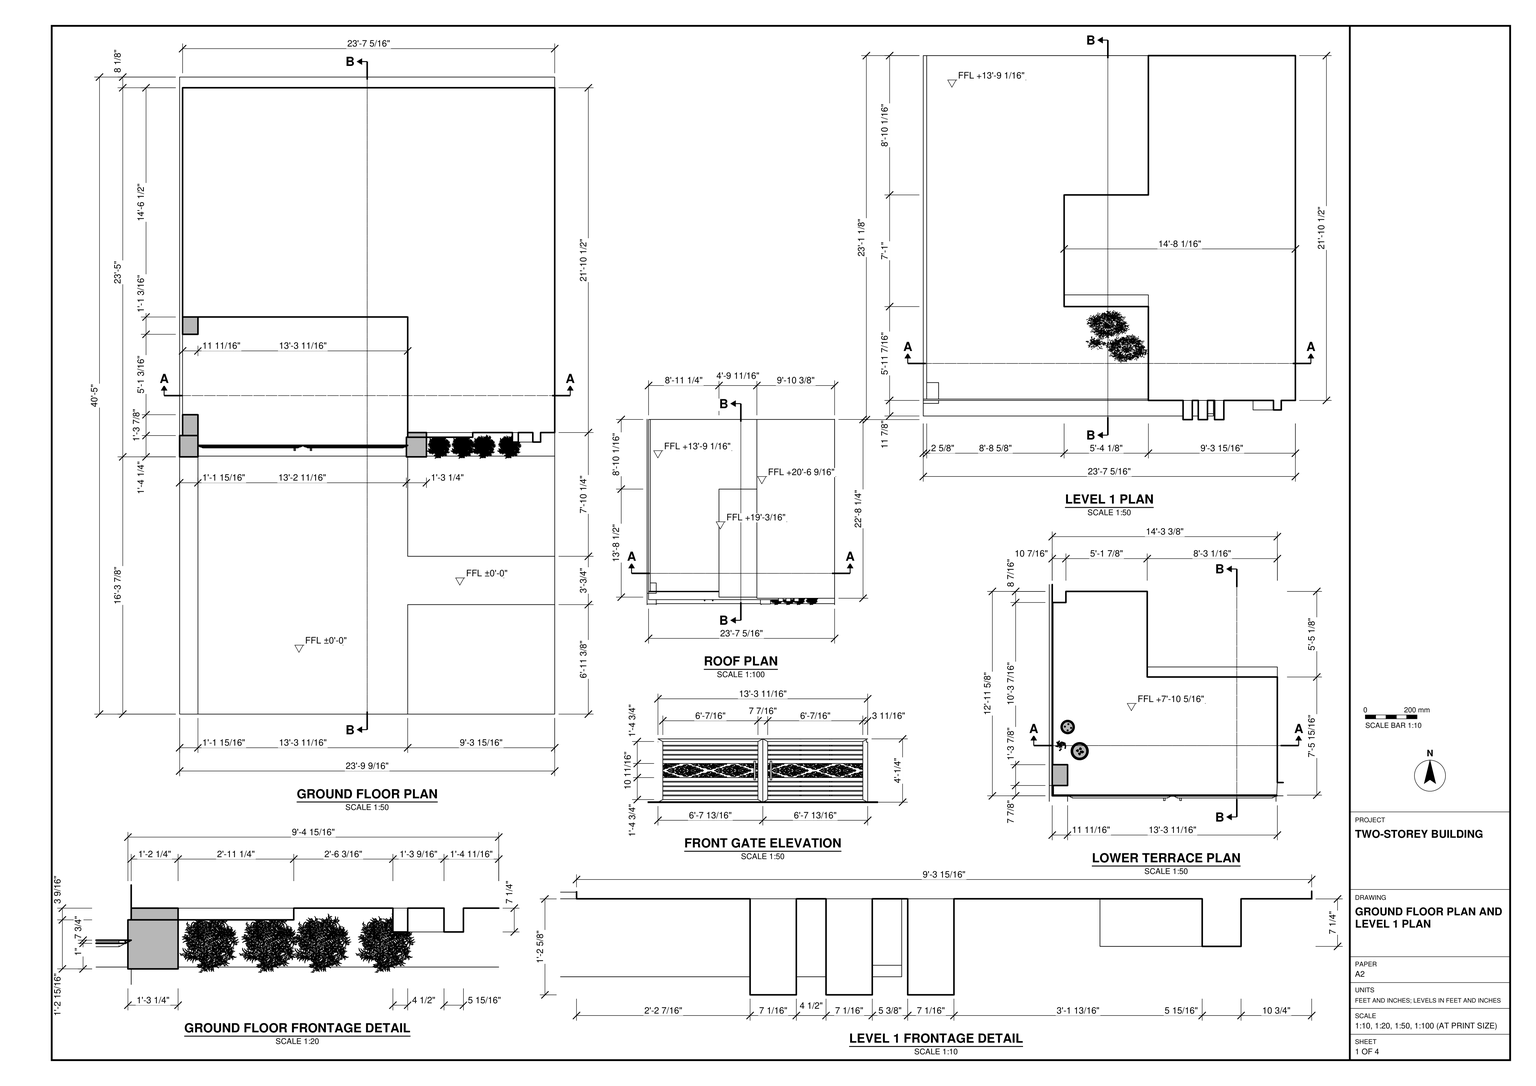
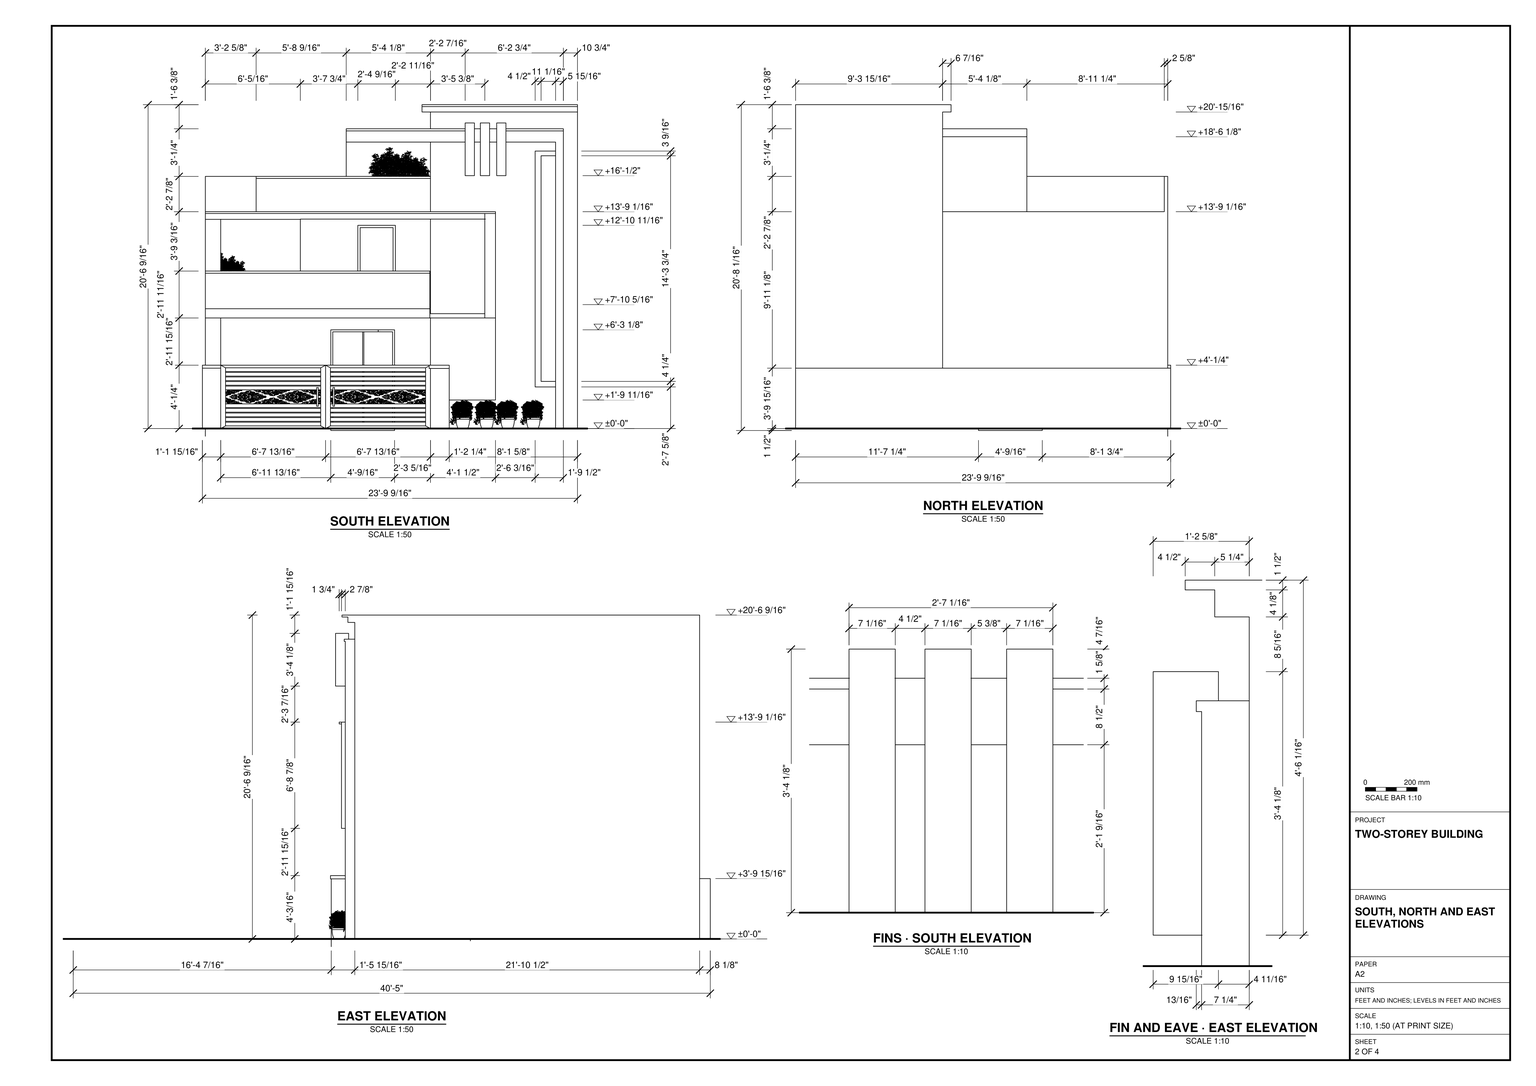
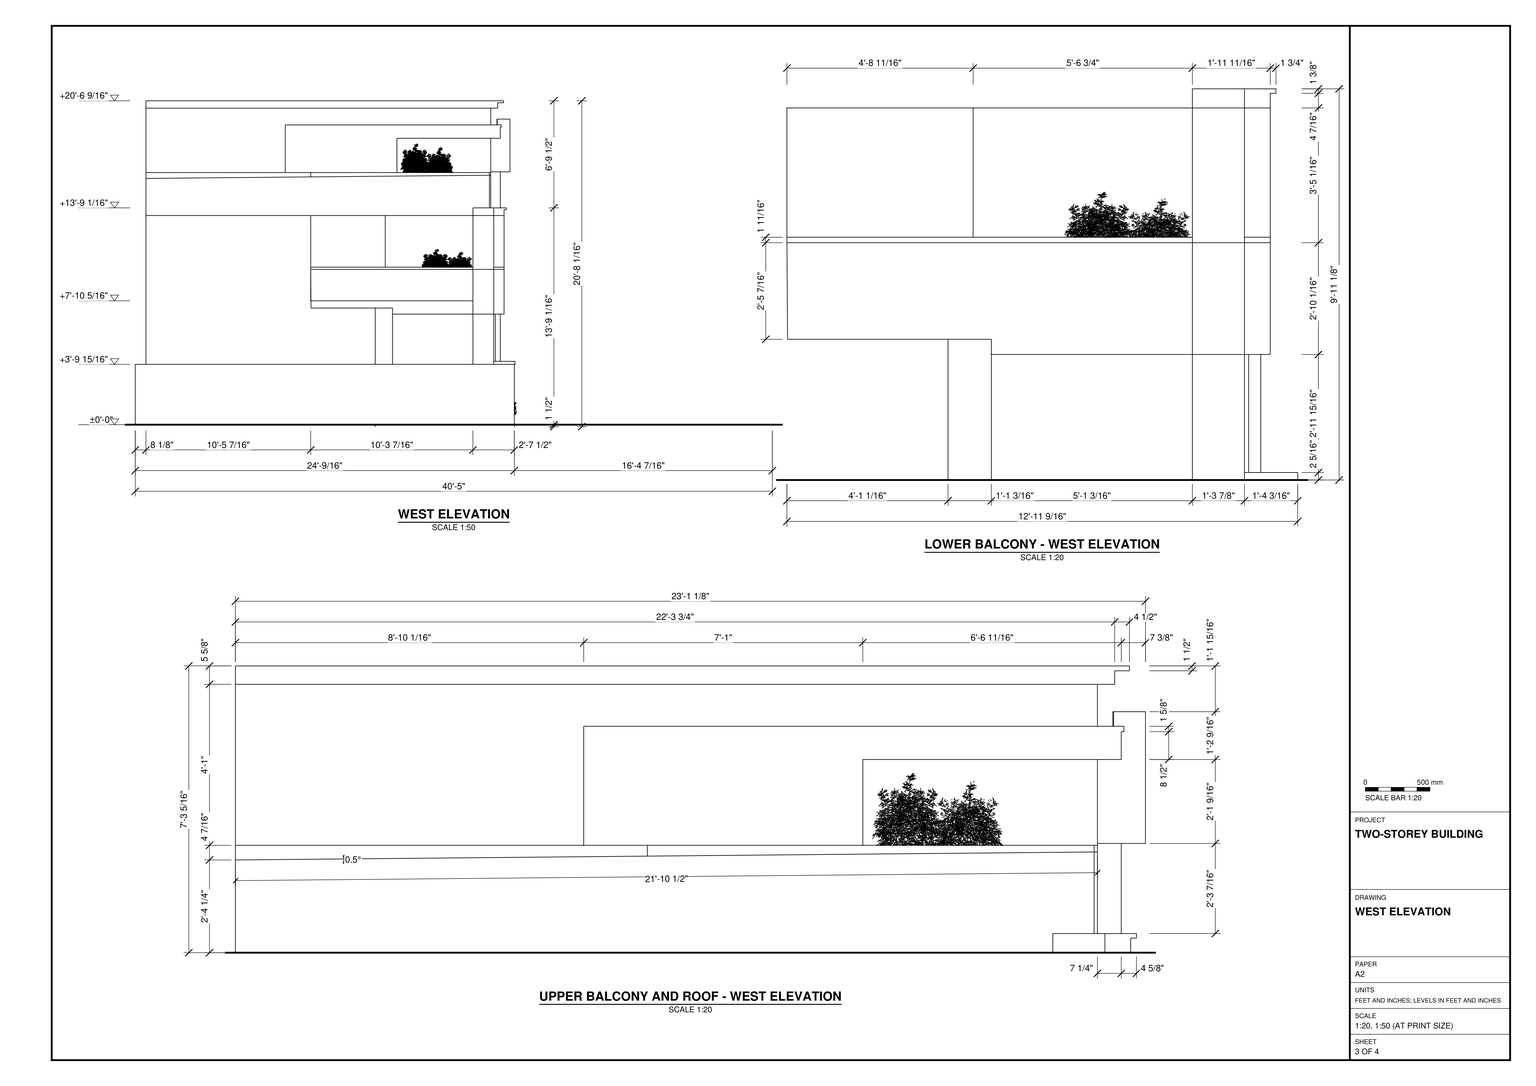
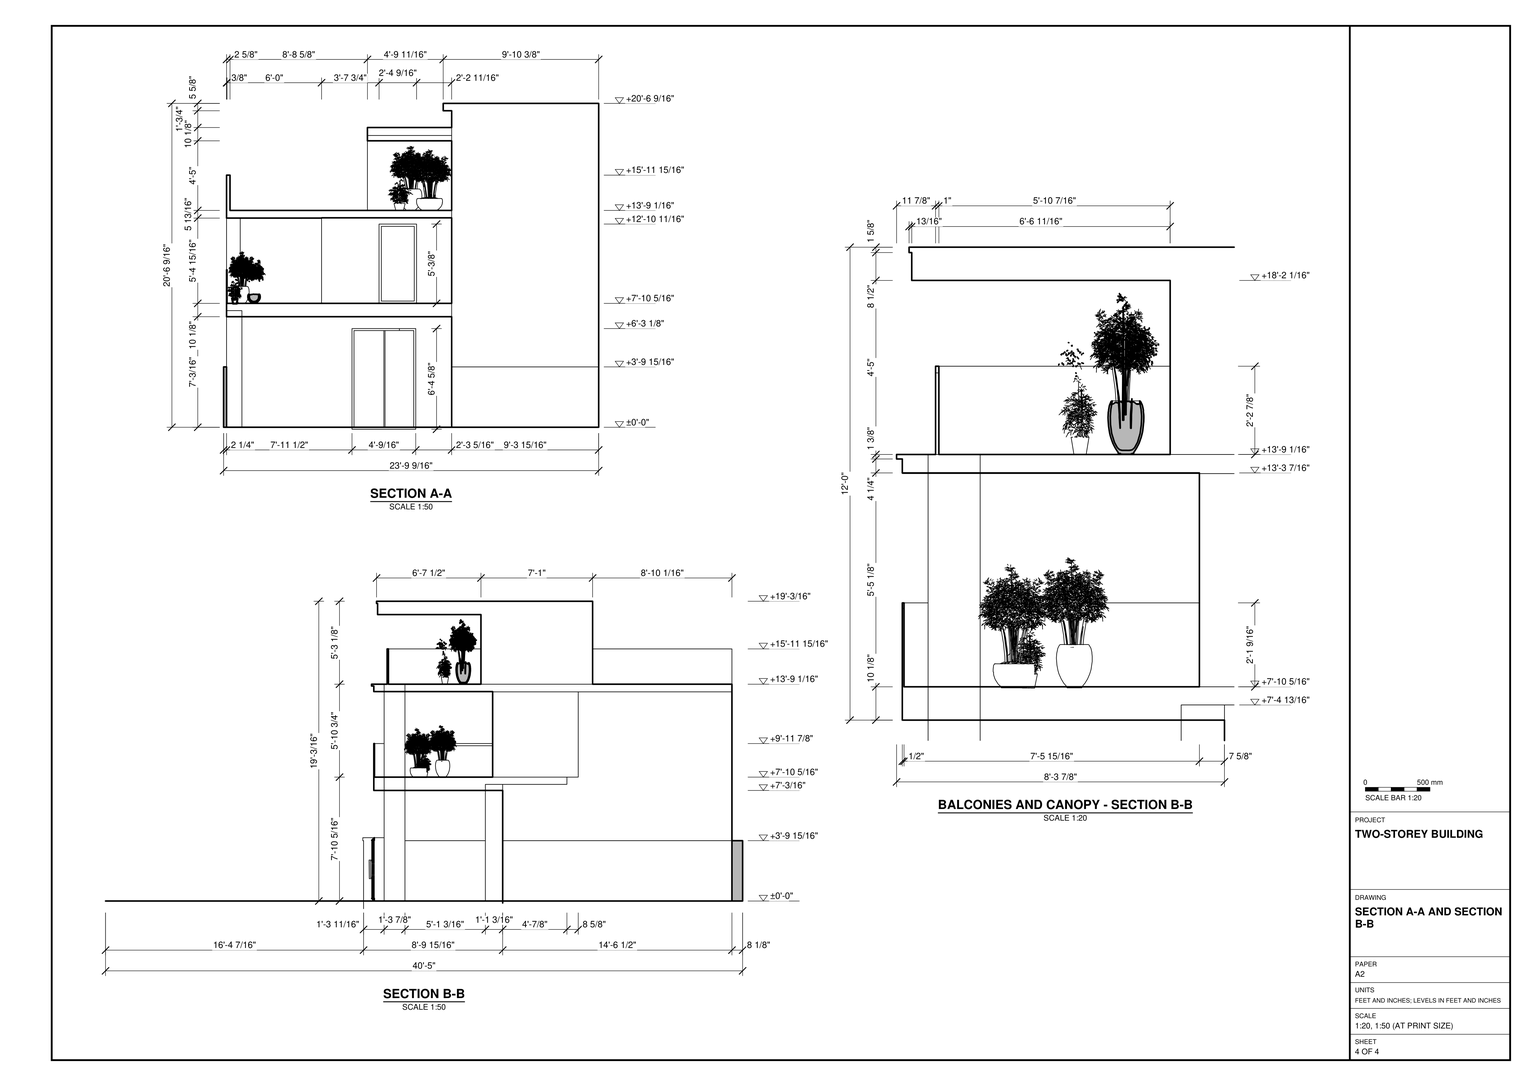
Build the two-storey building and its frontage in SketchUp from task_files/diagram_01.pdf. Work in feet and inches. Including the ground surface in front of the gate, the model must measure 23'-9 9/16" across the frontage, 40'-5" from front to back and 20'-8 1/16" in overall height. Set the ground floor at ±0'-0" and Level 1 at +13'-9 1/16". The lower terrace is between these levels at +7'-10 5/16".

Use the plans to set out the walls, openings, slab edges and terrace recesses. Follow the drawn thicknesses of the walls and parapets. On the south frontage, place the paired gate leaves between posts in front of the open bay, with the row of planters to the right. Use the west elevation to shape the solid balcony fronts and the setbacks between the terraces and flat roof planes. Include the tall frame on the right of the south elevation, its projecting eave and the three vertical fins.

Keep shell elements such as walls, slabs and roof pieces in separate groups or components, and group each furniture or joinery piece separately. Use components for repeated parts. Decor and loose items, including plants, may be any suitable library components. Save one SketchUp model as output_files/two_storey_building_stepped_terraces_and_gated_frontage.skp.

# SketchUp Ruby script. Lengths in inches.
U = 1.inch
M = Sketchup.active_model
def pt(a) = Geom::Point3d.new(a.map { |v| v * U })
def face(e, loops, mat)
  f = e.add_face(loops[0].map { |a| pt(a) })
  loops[1..].each { |l| e.add_face(l.map { |a| pt(a) }).erase! }
  f.material = f.back_material = mat if mat
  f
end
# faces: each face lists its corners as indices into pts; further lists are holes
def faces(e, pts, list, mat = nil) = list.each { |f| face(e, (f[0].is_a?(Array) ? f : [f]).map { |l| l.map { |i| pts[i] } }, mat) }
# xy, xz, yz: faces in a plane at the given z, y or x. An outline is a flat list of corners, or four numbers for a rectangle; further outlines are holes
def ring(l) = l.size == 4 ? [[l[0], l[1]], [l[2], l[1]], [l[2], l[3]], [l[0], l[3]]] : l.each_slice(2).to_a
def flat(e, list, mat, &to3) = list.each { |f| face(e, (f[0].is_a?(Array) ? f : [f]).map { |l| ring(l).map { |u, v| to3.(u, v) } }, mat) }
def xy(e, z, list, mat = nil) = flat(e, list, mat) { |x, y| [x, y, z] }
def xz(e, y, list, mat = nil) = flat(e, list, mat) { |x, z| [x, y, z] }
def yz(e, x, list, mat = nil) = flat(e, list, mat) { |y, z| [x, y, z] }
def lines(e, pts, list) = list.each { |a, b| e.add_line(pt(pts[a]), pt(pts[b])) }
# prism: a flat outline (further loops are holes) pulled along v
def prism(e, loops, v, mat = nil)
  f = face(e, loops, mat); d = Geom::Vector3d.new(v.map { |x| x * U })
  f.pushpull(f.normal.samedirection?(d) ? d.length : -d.length)
end
def box(e, o, s, mat = nil) = prism(e, [[o, [o[0] + s[0], o[1], o[2]], [o[0] + s[0], o[1] + s[1], o[2]], [o[0], o[1] + s[1], o[2]]]], [0, 0, s[2]], mat)
def at(x, y, z, deg = 0) = Geom::Transformation.translation(pt([x, y, z])) * Geom::Transformation.rotation(ORIGIN, Z_AXIS, deg.degrees)
def axes(o, x, y, z) = Geom::Transformation.new([*x, 0, *y, 0, *z, 0, *pt(o).to_a, 1])
def part(name) = M.definitions.add(name)
# library, detail: a bought-in or finely detailed component or shape, given as its bounding box
def library(name, o, s) = part(name).tap { |d| box(d.entities, o, s) }
def detail(e, o, s) = box(e.add_group.entities, o, s)
def put(e, d, t, mat = nil) = e.add_instance(d, t).tap { |i| i.material = mat if mat }
def group(e, t, mat = nil) = e.add_group.tap { |g| g.transformation = t; g.material = mat if mat }.entities
root = M.entities
M.materials.add("Material__2").color = [217, 199, 172]
M.materials.add("Material__3").color = [91, 133, 74]
M.materials.add("Material__4").color = [174, 125, 66]
M.materials.add("Niraj_Hair_Dark").color = [109, 109, 109]
M.materials.add("[0009_Linen]").color = [250, 240, 230]
M.materials.add("[Asphalt New]").color = [67, 60, 62]
M.materials.add("[Cladding Siding White]").color = [207, 207, 207]
M.materials.add("[Field Square Tile]").color = [217, 201, 169]
M.materials.add("[Grass Dark Green]").color = [106, 157, 55]
M.materials.add("[Polished Concrete New]").color = [200, 200, 203]
M.materials.add("[Translucent Glass Gray]").color = [128, 128, 128]
M.materials["[Translucent Glass Gray]"].alpha = 0.5
c1 = library("gate+(2)",[80.86,47.73,0.57],[129,4.01,72])
c2 = library("N_Plant_4",[-12.12,-0.17,0],[15.33,15.33,4.43])
c3 = library("Group\#1",[-35.09,50.53,0.35],[65,65.01,78.63])
c4 = library("Group\#3",[-47.79,-11.52,16.8],[25.3,23.96,12.71])
c5 = library("Group\#5",[-64.15,18.03,113.23],[126.13,128.06,125.3])
c6 = library("Group\#6",[-43.12,34.07,23.92],[89.16,89.66,208.68])
c7 = library("Group\#9",[-68.4,-38.23,21.61],[71.82,69.27,94.54])
c8 = library("Group\#2",[0,0,0],[52.97,53.78,94.24])
c9 = part("BAMBOO+PLANTS+18")
p = [[76.1,-18.67,124.1875],[75.64,-21.91,125.89],[75.32,-23.53,126.15],[59.79,-18.95,125.73],[59.73,-18.91,125.86],[59.71,-18.92,125.89],
  [73.4,-32.92,127.65],[74.6875,-27.4375,127.73],[63.89,-16.8125,129.85],[63.98,-16.98,129.67],[63.9,-16.93,129.65],[54.2,-40.02,131.12],
  [53.34,-40.74,130.4],[53.34,-40.76,130.39],[54.62,-40.88,131.27],[66.32,-27.13,131.12],[66.96,-28.05,130.4],[66.97,-28.05,130.39],
  [67.21,-26.79,131.27],[40.13,-26.8,131.12],[39.49,-25.88,130.4],[39.47,-25.875,130.39],[39.24,-27.14,131.27],[52.25,-13.91,131.12],
  [53.1,-13.18,130.4],[53.11,-13.17,130.39],[51.83,-13.05,131.27],[37.25,-9.43,132.85],[39.29,-8.57,132.36],[38.0625,-9.16,132.56],
  [39.79,-61.39,152.54],[39.7,-61.4,152.53],[39.71,-61.41,152.53],[86.35,-43.34,152.54],[86.35,-43.4375,152.53],[86.36,-43.43,152.53],
  [40.87,-34.12,153.87],[40.85,-34.17,153.85],[41.13,-35.3,153.74],[41.86,-33.73,154.33],[24.4375,-19.99,157.91],[25.55,-23.13,158.57],
  [26.09,-24.25,158.52],[26.98,-26.09,158.4375],[26.32,-24.85,158.6],[79.83,-48.03,159.18],[73.61,-53.28,162.3],[73.21,-53.58,162.4],
  [68.76,-56.92,163.58],[71.71,-54.84,163.13],[50.78,-53.31,168],[51.48,-52.9375,168.27],[53.15,-52.22,169.36],[0,0,0],
  [1,0,0],[1,1,0]]
faces(c9.entities,p,[[0,1,2],[3,4,5],[6,2,7],[8,9,10],[11,12,13,14],[15,16,17,18],[19,20,21,22],[23,24,25,26],
  [27,28,29],[30,31,32],[33,34,35],[36,37,38,39],[40,41,42],[43,42,44],[45,46,47],[48,47,49],
  [50,51,52]],"Material__3")
lines(c9.entities,p,[[53,54],[54,55],[55,53]])
put(c9.entities,c3,at(0,0,0))
put(c9.entities,c4,at(0,0,0),"Material__2")
g1 = group(c9.entities,at(0,0,0))
xy(g1,0.11,[[-40.33,-11.125,-46.1,4.71,-23.98,-4.79],[-40.33,-11.125,-23.98,-4.79,-39.85,-10.93],[-23.98,-4.79,-46.1,4.71,-29.74,11.03]])
xy(g1,2.33,[[-39.19,-8.96,-26.12,-4.19,-43.96,4.11],[-26.12,-4.19,-30.88,8.88,-43.96,4.11]])
p = [[-46.1,4.71,0.11],[-42.6,-16.26,25.42],[-51.25,7.53,25.42],[-40.33,-11.125,0.11],[-39.94,-11.2,0.39],[-24.0625,-5.39,0.19],
  [-39.85,-10.93,0.11],[-23.98,-4.79,0.11],[-27.47,16.18,25.42],[-18.82,-7.61,25.42],[-29.74,11.03,0.11],[-46.03,5.32,0.32],
  [-30.14,11.12,0.39],[-43.96,4.11,2.33],[-48.28,6.13,25.43],[-41.21,-13.28,25.43],[-39.19,-8.96,2.33],[-21.8,-6.21,25.43],
  [-26.12,-4.19,2.33],[-28.86,13.2,25.43],[-30.88,8.88,2.33]]
faces(g1,p,[[0,1,2],[0,3,1],[3,4,1],[4,3,5],[3,6,5],[5,6,7],[7,8,9],[9,5,7],
  [7,10,8],[11,0,2],[10,0,11],[12,10,11],[10,12,8],[4,5,9],[12,11,2],[4,9,1],
  [12,2,8],[13,14,15],[13,15,16],[16,15,17],[16,17,18],[18,17,19],[18,19,20],[20,14,13],
  [20,19,14],[2,1,15],[1,17,15],[1,9,17],[2,15,14],[9,19,17],[9,8,19],[8,2,14],
  [8,14,19]])
put(c9.entities,c5,at(0,0,0),"Material__3")
put(c9.entities,c6,at(0,0,0),"Material__4")
put(c9.entities,c7,at(0,0,0),"Material__3")
g2 = group(c9.entities,at(0,0,0),"Material__4")
p = [[-33.47,-3.44,22.53],[-32.52,-2.18,22.29],[-35,-2.42,22.52],[-32.63,-2.36,51.625],[-33.86,-0.87,22.51],[-32.99,-1.23,39.44],
  [-40.33,1.79,22.45],[-38.7,1.26,22.45],[-39.68,3.17,22.31],[-38.29,2.82,22.52],[-40.02,2.56,64.1875],[-38.96,2.96,67.41],
  [-32.67,3.09,22.4],[-32.78,4.75,22.31],[-33.97,3.49,22.47],[-32.22,3.72,37.36],[-33.99,3.83,35.86],[-32.76,4.76,35.15],
  [-39.5,1.15,36.98],[-38.21,2.29,38.55],[-33.09,3.04,35.25],[-34.77,-2.79,39.43],[-33.53,-3.3125,39.55],[-34.61,-1.32,39.42],
  [-32.42,3.27,34.95],[-27.02,-2.125,43.21],[-29.18,-0.11,39.05],[-32.83,4.3125,84.58],[-33.54,4.11,84.61],[-33,3.5,84.97],
  [-40.99,-3.99,40.53],[-37.78,-0.78,36.85],[-39.2,-2.22,37.99],[-39.87,1.72,66.76],[-38.69,1.58,66.95],[-38.26,2.14,37.47],
  [-34.27,1.66,40.3],[-37.98,1.99,37.24],[-34.66,1.75,40.37],[-33.97,-3.26,56.98],[-34.8,-1.93,56.8125],[-33.35,-1.15,56.73],
  [-39.16,-1.85,40.75],[-35.32,-1.95,39.66],[-39.13,-1.87,40.48],[-25.81,0.78,42.1],[-32.49,-1.74,39.66],[-25.4375,0.84,42.01],
  [-29.84,1.3,45.6],[-42.85,-1.89,41.97],[-42.87,-1.87,42.27],[-45.81,-1.85,43.9],[-22.74,1.83,43.89],[-36.07,4.4,44.34],
  [-38.34,10.67,54.83],[-38.22,10.32,54.68],[-33.35,-2.98,74.07],[-32.87,-1.8125,74.54],[-38.55,11.28,58.8],[-34.25,-1.41,81.65],
  [-34.0625,-2.71,108.29],[-29.24,2.34,63.78],[-33.29,-2.37,57.09],[-30.97,0.23,59.875],[-37.37,5.16,62.38],[-34.13,4.28,60.03],
  [-37.41,5.2,62.35],[-39.69,1.88,96.72],[-39.34,2.76,96.46],[-40.43,3.75,67.19],[-39.625,2.67,66.67],[-40.49,3.97,67.07],
  [-38.72,1.98,96.74],[-41.32,4.31,68.24],[-31.21,2.72,74.7],[-31.75,3.11,73.57],[-32.46,3.57,72.6],[-35.88,-5.78,75.21],
  [-35.14,-4.54,74.12],[-35.75,-5.44,74.67],[-33.08,-2.2,107.79],[-33.71,-1.51,108.28],[-38.53,1.82,81.89],[-35.87,0.98,82.73],
  [-38.52,1.875,81.92],[-39.97,4.35,96.9375],[-40.4375,5.01,98.17],[-38.98,2.88,95.9],[-38.86,2.5625,96.19],[-36.65,3.69,97.51],
  [-38.91,2.63,96.28],[-37.38,0.42,97.58],[-38.42,1.37,96.77],[-37.13,-0.07,98.07]]
faces(g2,p,[[0,1,2],[3,1,0],[2,1,4],[5,1,3],[1,5,4],[6,7,8],[7,9,8],[10,6,8],
  [10,8,11],[9,11,8],[12,13,14],[12,15,13],[13,16,14],[15,17,13],[16,13,17],[18,7,6],
  [19,7,18],[9,7,19],[20,12,14],[15,12,20],[21,0,2],[22,0,21],[3,0,22],[21,2,23],
  [23,2,4],[5,23,4],[18,6,10],[11,9,19],[16,20,14],[24,25,26],[15,27,17],[28,16,17],
  [17,27,28],[16,29,20],[15,20,29],[29,16,28],[30,31,32],[33,18,10],[34,18,33],[18,34,19],
  [35,36,37],[38,37,36],[38,35,37],[27,15,29],[35,38,36],[34,11,19],[39,21,40],[39,22,21],
  [23,40,21],[41,5,3],[23,41,40],[41,23,5],[22,39,3],[42,43,44],[45,46,47],[48,38,36],
  [42,44,49],[50,42,49],[51,50,49],[47,52,45],[53,54,55],[3,39,56],[57,3,56],[3,57,41],
  [58,55,54],[59,40,41],[57,59,41],[40,60,39],[60,40,59],[39,60,56],[61,62,63],[64,65,66],
  [10,67,33],[67,10,68],[68,10,11],[69,70,71],[33,67,34],[67,72,34],[34,72,11],[73,69,71],
  [68,11,72],[74,75,76],[77,78,79],[60,80,56],[80,57,56],[57,80,81],[59,57,81],[60,59,81],
  [82,83,84],[28,27,29],[85,86,87],[88,89,90],[67,68,72],[91,92,93],[80,60,81]],"Material__4")
put(c9.entities,c8,axes([-9.84,-90.99,0.24],[2.38095,0,0],[0,2.38095,0],[0,0,2.38095]))
xy(root,0,[[0,196.43,2.25,196.43,2.25,212.09,13.9375,212.09,13.9375,227.95,2.25,227.95,2.25,289.15,13.9375,289.15,13.9375,302.34,2.25,302.34,2.25,476.86,285.53,476.86,285.53,484.99,0,484.99],[2.25,196.43,13.9375,212.09],[173.61,196.43,187.89,214.36]])
xy(root,0,[[268.86,207.11,274.78,207.11,274.78,214.36,285.53,214.36,285.53,476.86,2.25,476.86,2.25,302.34,173.61,302.34,173.61,214.36,268.86,214.36]],"[Field Square Tile]")
xy(root,0,[[0,0,13.9375,196.43],[173.61,0,285.53,83.375],[173.61,120.14,285.53,196.43],[187.89,196.43,285.53,196.43,285.53,214.36,274.78,214.36,274.78,207.11,268.86,207.11,268.86,214.36,187.89,214.36]],"[Grass Dark Green]")
xy(root,0,[[13.9375,0,173.61,0,173.61,83.375,285.53,83.375,285.53,120.14,173.61,120.14,173.61,196.43,13.9375,196.43],[13.9375,196.43,173.61,196.43,173.61,302.34,13.9375,302.34,13.9375,289.15,2.25,289.15,2.25,227.95,13.9375,227.95]],"[Polished Concrete New]")
xy(root,21.7,[[173.61,210.8,223.11,214.36]])
xy(root,31.65,[[253.3,207.11,268.86,214.36]])
xy(root,35.88,[[257.8125,207.11,268.86,214.36]])
xy(root,45.72,[[172.61,195.86,187.89,196.43],[172.61,196.43,173.61,210.8]])
xy(root,45.9375,[[0,195.86,2.25,196.43],[2.25,195.86,13.9375,196.43],[0,196.43,2.25,212.09],[0,212.09,2.25,212.09,2.25,476.86,285.53,476.86,285.53,484.99,0,484.99]])
xy(root,48.22,[[0,195.86,13.9375,212.09],[172.61,195.86,187.89,195.86,187.89,214.36,173.61,214.36,173.61,210.8,172.61,210.8]])
xy(root,84.17,[[2.25,204.24,2.25,289.15,13.9375,289.15,13.9375,302.34,173.61,302.34,173.61,210.8,223.11,210.8,223.11,204.24]],"[0009_Linen]")
xy(root,87.4375,[[173.16,204.24,214.99,204.24,215.45,214.36,173.61,214.36]])
xy(root,94.3125,[[173.16,204.24,173.18,204.24,173.18,204.76],[2.96,204.76,173.18,204.76,173.61,214.36,173.61,294.7,74.57,294.7,74.57,359.85,12.66,359.85,12.66,351.42,2.6,351.42,2.6,227.95,13.9375,227.95,13.9375,212.09,2.96,212.09]])
xy(root,119.875,[[2.25,204.24,173.16,204.24,173.18,204.76,2.96,204.76,2.96,212.09,2.25,212.09],[2.25,227.95,2.6,351.42]])
xy(root,159.24,[[2.25,204.24,2.25,351.42,12.66,351.42,12.66,359.85,74.57,359.85,74.57,204.24]],"[0009_Linen]")
xy(root,159.44,[[74.57,204.24,74.57,294.7,173.61,294.7,173.61,214.36,215.45,214.36,215.45,204.24]],"[0009_Linen]")
xy(root,163.69,[[2.25,202.49,223.11,204.24]])
xy(root,165.0625,[[2.25,202.49,223.11,202.49,223.11,204.24,214.99,204.24,215.17,208.11,215.45,214.36,13.9375,214.36,13.9375,212.09,2.25,212.09],[214.99,204.24,223.11,204.24,223.11,214.36,215.45,214.36,215.17,208.11],[2.25,212.09,13.9375,214.36],[2.25,214.36,13.9375,215.37],[2.25,215.37,4.88,227.95],
  [13.9375,215.37,173.61,215.37,173.61,285.8,109.49,285.8,109.49,370.8,173.61,370.8,173.61,476.86,4.88,476.86,4.88,227.95,13.9375,227.95],[4.88,215.37,13.9375,227.95]])
xy(root,191.9375,[[2.25,214.36,173.61,215.37]])
xy(root,191.9375,[[2.25,215.37,4.88,476.86]],"Niraj_Hair_Dark")
xy(root,192.5,[[200.03,199.74,207.07,214.36],[211.59,199.74,218.63,214.36],[224.03,199.74,231.07,214.36]])
xy(root,207.64,[[257.8125,207.11,268.86,214.36]])
xy(root,211.22,[[253.3,207.11,268.86,214.36]])
xy(root,218.07,[[207.07,207.11,211.59,214.36],[218.63,207.11,224.03,214.36],[231.07,207.11,268.86,214.36]])
xy(root,218.07,[[109.49,207.11,109.49,285.8,173.61,285.8,173.61,214.36,200.03,214.36,200.03,207.11]],"[0009_Linen]")
xy(root,226.55,[[109.49,206.3,200.03,207.11],[231.07,206.3,274.78,207.11]],"[0009_Linen]")
xy(root,228.19,[[109.49,206.3,200.03,206.3,200.03,209.43,207.07,209.43,207.07,207.11,211.59,207.11,211.59,209.11,218.63,209.11,218.63,207.11,224.03,207.11,224.03,209.68,231.07,209.68,231.07,206.3,274.78,206.3,274.78,214.36,173.61,214.36,173.61,370.8,109.49,370.8]])
xy(root,232.63,[[200.03,199.74,207.07,209.43],[211.59,199.74,218.63,209.11],[224.03,199.74,231.07,209.68]])
xy(root,240.96,[[173.61,209.11,285.53,214.36]])
xy(root,240.96,[[167.17,209.11,173.61,476.86]],"[0009_Linen]")
xy(root,245.08,[[167.17,204.61,285.53,209.11]],"[0009_Linen]")
xy(root,246.5625,[[167.17,204.61,285.53,476.86]])
xz(root,195.86,[[172.61,45.72,187.89,48.22],[0,45.9375,13.9375,48.22]])
xz(root,196.43,[[0,0,13.9375,45.9375],[173.61,0,187.89,45.72]])
xz(root,199.74,[[200.03,192.5,207.07,232.63],[211.59,192.5,218.63,232.63],[224.03,192.5,231.07,232.63]])
xz(root,202.49,[[2.25,163.69,223.11,165.0625]],"[0009_Linen]")
xz(root,204.24,[[173.16,84.17,214.99,87.4375],[2.25,118.2,173.16,119.875],[214.99,163.69,223.11,165.0625]])
xz(root,204.24,[[2.25,84.17,173.16,91.1875],[214.99,84.17,223.11,163.69],[2.25,159.24,74.57,159.24,74.57,159.44,214.99,159.44,214.99,163.69,2.25,163.69]],"[0009_Linen]")
xz(root,204.24,[[2.25,91.1875,173.16,118.2]],"[Translucent Glass Gray]")
xz(root,204.61,[[167.17,245.08,285.53,246.5625]],"[0009_Linen]")
xz(root,204.76,[[2.96,94.3125,173.18,119.875]],"[Translucent Glass Gray]")
xz(root,206.3,[[109.49,226.55,200.03,228.19],[231.07,226.55,274.78,228.19]],"[0009_Linen]")
xz(root,207.11,[[268.86,0,274.78,0,274.78,226.55,231.07,226.55,231.07,218.07,268.86,218.07],[253.3,31.65,268.86,31.65,268.86,35.88,257.8125,35.88,257.8125,207.64,268.86,207.64,268.86,211.22,253.3,211.22],[109.49,218.07,200.03,226.55],[207.07,218.07,211.59,228.19],[218.63,218.07,224.03,228.19]],"[0009_Linen]")
xz(root,209.11,[[211.59,228.19,218.63,232.63]])
xz(root,209.11,[[167.17,240.96,285.53,245.08]],"[0009_Linen]")
xz(root,209.43,[[200.03,228.19,207.07,232.63]])
xz(root,209.68,[[224.03,228.19,231.07,232.63]])
xz(root,210.8,[[172.61,45.72,173.61,48.22]])
xz(root,210.8,[[173.61,21.7,223.11,84.17]],"[Cladding Siding White]")
xz(root,212.09,[[2.25,0,13.9375,48.22],[0,45.9375,2.25,48.22]])
xz(root,212.09,[[2.25,48.22,13.9375,94.3125],[2.96,94.3125,13.9375,94.3125,13.9375,165.0625,2.25,165.0625,2.25,119.875,2.96,119.875]],"[0009_Linen]")
xz(root,214.36,[[173.61,0,187.89,21.7],[187.89,0,268.86,0,268.86,31.65,253.3,31.65,253.3,211.22,268.86,211.22,268.86,218.07,231.07,218.07,231.07,192.5,224.03,192.5,224.03,218.07,218.63,218.07,218.63,192.5,211.59,192.5,211.59,218.07,207.07,218.07,207.07,192.5,200.03,192.5,200.03,218.07,173.61,218.07,173.61,165.0625,223.11,165.0625,223.11,21.7,187.89,21.7],[274.78,0,285.53,0,285.53,240.96,173.61,240.96,173.61,228.19,274.78,228.19],[173.61,21.7,187.89,48.22],[173.61,87.4375,215.45,159.44],
  [2.25,165.0625,40.9,191.9375],[40.9,190.375,173.61,191.9375]])
xz(root,214.36,[[257.8125,35.88,268.86,207.64],[40.9,165.0625,173.61,190.375]],"[Translucent Glass Gray]")
xz(root,215.37,[[4.88,165.0625,173.61,191.9375]],"[Translucent Glass Gray]")
xz(root,227.95,[[2.25,0,2.25,119.875,2.6,119.875,2.6,94.3125,13.9375,94.3125,13.9375,0],[2.6,94.3125,2.6,119.875,2.25,119.875,2.25,165.0625,13.9375,165.0625,13.9375,94.3125]])
xz(root,285.8,[[109.49,165.0625,173.61,218.07]])
xz(root,289.15,[[2.25,0,13.9375,84.17]])
xz(root,294.7,[[74.57,94.3125,118.33,94.3125,118.33,154.6875,146.89,154.6875,146.89,94.3125,173.61,94.3125,173.61,159.44,74.57,159.44]])
xz(root,294.7,[[[118.33,94.3125,146.89,154.6875],[120.08,96.06,145.15,152.94]]],"[Asphalt New]")
xz(root,294.7,[[120.08,96.06,145.15,152.94]],"[Translucent Glass Gray]")
xz(root,302.34,[[97.74,-1.52,146.27,0],[2.25,0,13.9375,88.79],[13.9375,0,97.74,0,97.74,75.14,146.27,75.14,146.27,0,173.61,0,173.61,84.17,13.9375,84.17]])
xz(root,302.34,[[97.74,0,99.26,0,99.26,73.62,133.83,73.62,133.83,75.14,97.74,75.14],[122.01,0,122.9,73.62],[144.76,0,146.27,0,146.27,75.14,133.83,75.14,133.83,73.62,144.76,73.62]],"[Asphalt New]")
xz(root,302.34,[[99.26,0,122.01,73.62],[122.9,0,144.76,73.62]],"[Translucent Glass Gray]")
xz(root,351.42,[[2.6,94.3125,12.66,94.3125,12.66,159.24,2.25,159.24,2.25,119.875,2.6,119.875]])
xz(root,359.85,[[12.66,94.3125,74.57,159.24]])
xz(root,370.8,[[109.49,165.0625,173.61,222.13],[109.49,222.13,173.61,228.19]])
xz(root,476.86,[[173.61,0,285.53,45.9375],[173.61,45.9375,173.61,240.96,167.17,240.96,167.17,246.5625,285.53,246.5625,285.53,45.9375]])
xz(root,476.86,[[2.25,0,173.61,45.9375],[2.25,45.9375,2.25,191.9375,4.88,191.9375,4.88,165.0625,173.61,165.0625,173.61,45.9375]],"[0009_Linen]")
xz(root,484.99,[[0,0,285.53,45.9375]])
yz(root,0,[[195.86,45.9375,212.09,48.22]])
yz(root,0,[[196.43,0,484.99,45.9375]],"[0009_Linen]")
yz(root,2.25,[[227.95,0,289.15,45.9375],[302.34,0,476.86,45.9375],[204.24,84.17,212.09,118.2],[212.09,84.17,227.95,118.2],[204.24,118.2,212.09,119.875],
  [227.95,118.2,227.95,119.875,351.42,119.875,351.4,118.2],[214.36,165.0625,214.36,189.92,215.37,189.91,215.37,165.0625],[215.37,189.91,214.36,189.92,214.36,191.9375,215.37,191.9375]])
yz(root,2.25,[[476.86,187.49,351.42,188.65,351.42,191.9375,476.86,191.9375],[351.42,188.65,215.37,189.91,215.37,191.9375,351.42,191.9375]],"Niraj_Hair_Dark")
yz(root,2.25,[[212.09,45.9375,227.95,84.17],[289.15,45.9375,302.34,88.79],[302.34,45.9375,302.34,88.79,351.22,88.79,351.4,118.2,351.42,119.875,351.42,159.24,476.86,159.24,476.86,45.9375],[227.95,84.17,227.95,118.2,351.4,118.2,351.22,88.79,289.15,88.79,289.15,84.17],[212.09,118.2,227.95,159.24],
  [204.24,159.24,204.24,163.69,202.49,163.69,202.49,165.0625,212.09,165.0625,212.09,159.24],[212.09,159.24,227.95,165.0625]],"[0009_Linen]")
yz(root,2.25,[[227.95,159.24,227.95,165.0625,215.37,165.0625,215.37,189.91,351.42,188.65,476.86,187.49,476.86,159.24]],"[Translucent Glass Gray]")
yz(root,2.6,[[227.95,94.3125,351.42,119.875]])
yz(root,2.96,[[204.76,94.3125,212.09,119.875]])
yz(root,4.88,[[215.37,165.0625,476.86,191.9375]],"[Translucent Glass Gray]")
yz(root,12.66,[[351.42,94.3125,359.85,159.24]])
yz(root,13.9375,[[196.43,0,212.09,0,212.09,48.22,195.86,48.22,195.86,45.9375,196.43,45.9375],[212.09,0,227.95,94.3125],[289.15,0,302.34,84.17],[212.09,94.3125,227.95,165.0625]])
yz(root,74.57,[[294.7,94.3125,359.85,159.24],[204.24,159.24,294.7,159.44]])
yz(root,109.49,[[285.8,165.0625,285.8,218.07,207.11,218.07,207.11,226.55,206.3,226.55,206.3,228.19,370.8,228.19,370.8,165.0625]])
yz(root,167.17,[[209.11,240.96,209.11,245.08,204.61,245.08,204.61,246.5625,476.86,246.5625,476.86,240.96]],"[0009_Linen]")
yz(root,172.61,[[195.86,45.72,210.8,48.22]])
yz(root,173.61,[[196.43,0,196.43,45.72,210.8,45.72,210.8,21.7,214.36,21.7,214.36,0],[210.8,21.7,214.36,48.22],[214.36,94.3125,294.7,159.44],[370.8,165.0625,370.8,228.19,214.36,228.19,214.36,240.96,476.86,240.96,476.86,165.0625]])
yz(root,173.61,[[214.36,0,214.36,48.22,210.8,48.22,210.8,84.17,302.34,84.17,302.34,0],[215.37,165.0625,215.37,191.9375,214.36,191.9375,214.36,218.07,285.8,218.07,285.8,165.0625]],"[0009_Linen]")
yz(root,187.89,[[196.43,0,214.36,0,214.36,48.22,195.86,48.22,195.86,45.72,196.43,45.72]])
yz(root,200.03,[[199.74,192.5,199.74,232.63,209.43,232.63,209.43,228.19,206.3,228.19,206.3,226.55,207.11,226.55,207.11,218.07,214.36,218.07,214.36,192.5]])
yz(root,207.07,[[199.74,192.5,214.36,192.5,214.36,218.07,207.11,218.07,207.11,228.19,209.43,228.19,209.43,232.63,199.74,232.63]])
yz(root,211.59,[[199.74,192.5,199.74,232.63,209.11,232.63,209.11,228.19,207.11,228.19,207.11,218.07,214.36,218.07,214.36,192.5]])
yz(root,218.63,[[199.74,192.5,214.36,192.5,214.36,218.07,207.11,218.07,207.11,228.19,209.11,228.19,209.11,232.63,199.74,232.63]])
yz(root,223.11,[[210.8,21.7,214.36,88.79],[204.24,84.17,210.8,84.17,210.8,88.79,214.36,88.79,214.36,165.0625,204.24,165.0625],[202.49,163.69,204.24,165.0625]])
yz(root,224.03,[[199.74,192.5,199.74,232.63,209.68,232.63,209.68,228.19,207.11,228.19,207.11,218.07,214.36,218.07,214.36,192.5]])
yz(root,231.07,[[199.74,192.5,214.36,192.5,214.36,218.07,207.11,218.07,207.11,226.55,206.3,226.55,206.3,228.19,209.68,228.19,209.68,232.63,199.74,232.63]])
yz(root,253.3,[[207.11,31.65,214.36,211.22]],"[0009_Linen]")
yz(root,257.8125,[[207.11,35.88,214.36,207.64]])
yz(root,268.86,[[207.11,0,214.36,31.65],[207.11,31.65,214.36,35.88],[207.11,35.88,214.36,207.64],[207.11,211.22,214.36,218.07]])
yz(root,274.78,[[207.11,0,214.36,0,214.36,228.19,206.3,228.19,206.3,226.55,207.11,226.55]])
yz(root,285.53,[[214.36,0,476.86,0,476.86,246.5625,204.61,246.5625,204.61,245.08,209.11,245.08,209.11,240.96,214.36,240.96],[476.86,0,484.99,45.9375]])
p = [[173.18,204.76,94.3125],[173.16,204.24,94.3125],[173.16,204.24,91.1875],[173.16,204.24,87.4375],[173.61,214.36,87.4375],[173.61,214.36,94.3125],
  [214.99,204.24,165.0625],[215.17,208.11,165.0625],[215.45,214.36,165.0625],[215.45,214.36,159.44],[215.45,214.36,87.4375],[214.99,204.24,87.4375],
  [214.99,204.24,159.44],[214.99,204.24,163.69],[173.18,204.76,119.875],[173.16,204.24,119.875],[173.16,204.24,118.2],[215.45,208.11,165.0625],
  [215.45,208.11,159.44],[187.89,196.43,45.72],[187.89,210.8,45.72],[173.61,370.8,222.13],[173.61,285.8,222.13],[109.49,285.8,222.13],
  [173.61,285.8,218.07],[2.25,196.43,-5.9],[2.25,196.43,0]]
faces(root,p,[[0,1,2,3,4,5],[6,7,8,9,10,11,12,13],[1,0,14,15,16]])
lines(root,p,[[17,18],[7,17],[19,20],[21,22],[23,22],[22,24],[25,26]])
put(root,c1,axes([-86.15,152.875,-0.38],[1.23778,0,0],[0,1,0],[0,0,0.6697]))
put(root,c2,axes([210.41,181.59,0],[2.856,0,0],[0,2.904,0],[0,0,4.89514]))
put(root,c2,axes([228.53,181.59,0],[2.856,0,0],[0,2.904,0],[0,0,4.89514]))
put(root,c2,axes([244.53,181.59,0],[2.856,0,0],[0,2.904,0],[0,0,4.89514]))
put(root,c2,axes([264.01,181.59,0],[2.856,0,0],[0,2.904,0],[0,0,4.89514]))
put(root,c9,axes([14.43,242.66,93.92],[0.168,0,0],[0,0.168,0],[0,0,0.168]))
put(root,c9,axes([143.14,258.36,165.0625],[0.26205,0,0],[0,0.168,0],[0,0,0.20664]))
